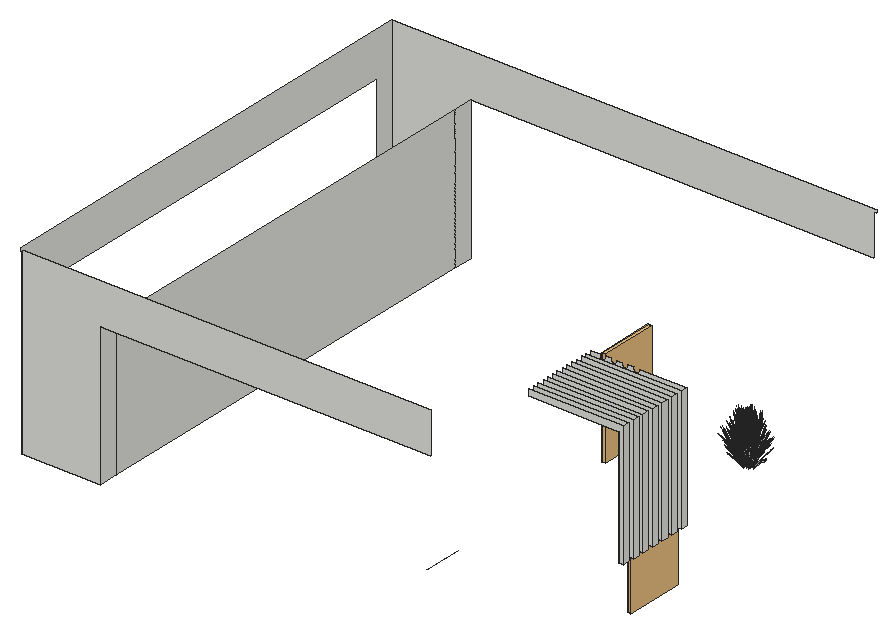
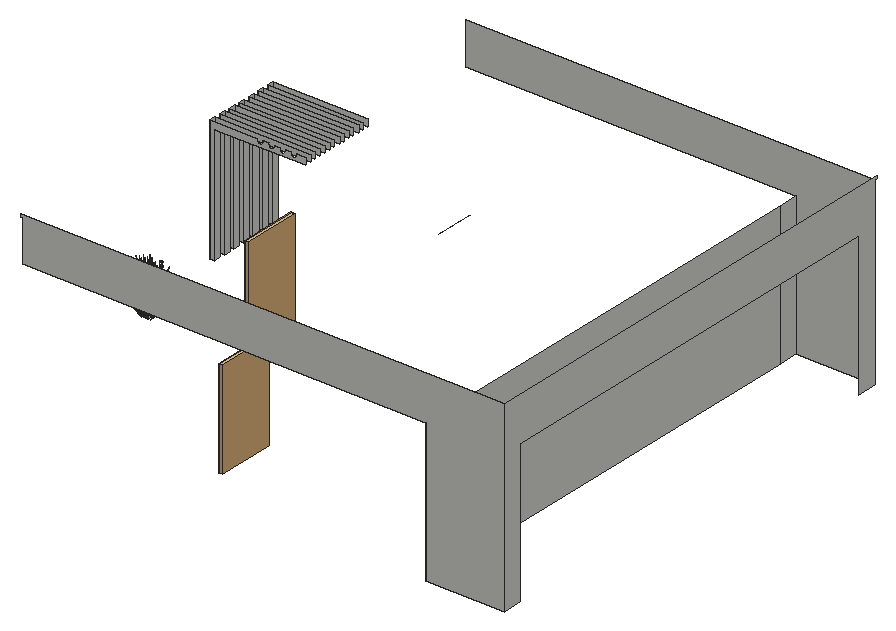
# SketchUp Ruby script. Lengths in millimetres.
U = 1.mm
M = Sketchup.active_model
def pt(a) = Geom::Point3d.new(a.map { |v| v * U })
def face(e, loops, mat)
  f = e.add_face(loops[0].map { |a| pt(a) })
  loops[1..].each { |l| e.add_face(l.map { |a| pt(a) }).erase! }
  f.material = f.back_material = mat if mat
  f
end
# faces: each face lists its corners as indices into pts; further lists are holes
def faces(e, pts, list, mat = nil) = list.each { |f| face(e, (f[0].is_a?(Array) ? f : [f]).map { |l| l.map { |i| pts[i] } }, mat) }
# xy, xz, yz: faces in a plane at the given z, y or x. An outline is a flat list of corners, or four numbers for a rectangle; further outlines are holes
def ring(l) = l.size == 4 ? [[l[0], l[1]], [l[2], l[1]], [l[2], l[3]], [l[0], l[3]]] : l.each_slice(2).to_a
def flat(e, list, mat, &to3) = list.each { |f| face(e, (f[0].is_a?(Array) ? f : [f]).map { |l| ring(l).map { |u, v| to3.(u, v) } }, mat) }
def xy(e, z, list, mat = nil) = flat(e, list, mat) { |x, y| [x, y, z] }
def xz(e, y, list, mat = nil) = flat(e, list, mat) { |x, z| [x, y, z] }
def yz(e, x, list, mat = nil) = flat(e, list, mat) { |y, z| [x, y, z] }
def lines(e, pts, list) = list.each { |a, b| e.add_line(pt(pts[a]), pt(pts[b])) }
# prism: a flat outline (further loops are holes) pulled along v
def prism(e, loops, v, mat = nil)
  f = face(e, loops, mat); d = Geom::Vector3d.new(v.map { |x| x * U })
  f.pushpull(f.normal.samedirection?(d) ? d.length : -d.length)
end
def box(e, o, s, mat = nil) = prism(e, [[o, [o[0] + s[0], o[1], o[2]], [o[0] + s[0], o[1] + s[1], o[2]], [o[0], o[1] + s[1], o[2]]]], [0, 0, s[2]], mat)
def at(x, y, z, deg = 0) = Geom::Transformation.translation(pt([x, y, z])) * Geom::Transformation.rotation(ORIGIN, Z_AXIS, deg.degrees)
def axes(o, x, y, z) = Geom::Transformation.new([*x, 0, *y, 0, *z, 0, *pt(o).to_a, 1])
def part(name) = M.definitions.add(name)
# library, detail: a bought-in or finely detailed component or shape, given as its bounding box
def library(name, o, s) = part(name).tap { |d| box(d.entities, o, s) }
def detail(e, o, s) = box(e.add_group.entities, o, s)
def put(e, d, t, mat = nil) = e.add_instance(d, t).tap { |i| i.material = mat if mat }
def group(e, t, mat = nil) = e.add_group.tap { |g| g.transformation = t; g.material = mat if mat }.entities
root = M.entities
M.materials.add("LightPink_Translucent").color = [144, 107, 117]
M.materials["LightPink_Translucent"].alpha = 0.8
c1 = library("porta+4",[5.1,-137.5,33.9],[1182.3,119.8,2113.3])
c2 = part("blade")
p = [[54.7,5.3,558.8],[0,4.4,0],[2.3,11.5,0],[55.5,7.8,558.8],[58.2,7.8,558.8],[9.8,11.5,0],
  [62.9,5.7,838.2],[63,6,838.2],[63.4,6,838.2]]
faces(c2.entities,p,[[0,1,2,3],[4,5,2,3],[6,0,3,7],[7,3,4,8]])
c3 = part("seeds")
p = [[7.6,-2.7,35.1],[-0.2,-0.6,40.4],[-0.2,-0.8,0.9],[3.5,-1.8,-1.7],[7.5,-0.8,76.3],[3.7,0.2,78.9]]
faces(c3.entities,p,[[0,1,2,3],[1,0,4,5]],"LightPink_Translucent")
c4 = part("blade with seeds")
put(c4.entities,c2,at(0,0,0))
put(c4.entities,c3,axes([60.9,6.5,787.2],[1.5799,-0.05474,1.17369],[-0.12525,1.92788,0.29478],[-0.07173,-0.02425,1.56792]))
xy(root,8077.2,[[16840.2,7010.7,16992.6,7213.9],[16840.2,7383.7,16992.6,7586.9],[16840.2,7756.7,16992.6,7959.9],[16840.2,8129.7,16992.6,8332.9],[16840.2,8502.7,16992.6,8705.9],
  [16840.2,8875.6,16992.6,9078.8],[16840.2,9248.6,16992.6,9449.1]])
xz(root,3200.4,[[1295.4,7315.2,3733.8,7315.2,3733.8,11734.8,14020.8,11734.8,14020.8,13030.2,1295.4,13030.2]])
xz(root,7010.7,[[16840.2,8077.2,16992.6,8077.2,16992.6,11938,14020.8,11938,14020.8,11734.8,16840.2,11734.8]])
xz(root,7213.9,[[16840.2,8077.2,16840.2,11734.8,14020.8,11734.8,14020.8,11938,16992.6,11938,16992.6,8077.2]])
xz(root,7383.7,[[16840.2,8077.2,16992.6,8077.2,16992.6,11938,14020.8,11938,14020.8,11734.8,16840.2,11734.8]])
xz(root,7586.9,[[16840.2,8077.2,16840.2,11734.8,14020.8,11734.8,14020.8,11938,16992.6,11938,16992.6,8077.2]])
xz(root,7756.7,[[16840.2,8077.2,16992.6,8077.2,16992.6,11938,14020.8,11938,14020.8,11734.8,16840.2,11734.8]])
xz(root,7959.9,[[16840.2,8077.2,16840.2,11734.8,14020.8,11734.8,14020.8,11938,16992.6,11938,16992.6,8077.2]])
xz(root,8129.7,[[16840.2,8077.2,16992.6,8077.2,16992.6,11938,14020.8,11938,14020.8,11734.8,16840.2,11734.8]])
xz(root,8332.9,[[16840.2,8077.2,16840.2,11734.8,14020.8,11734.8,14020.8,11938,16992.6,11938,16992.6,8077.2]])
xz(root,8502.7,[[16840.2,8077.2,16992.6,8077.2,16992.6,11938,14020.8,11938,14020.8,11734.8,16840.2,11734.8]])
xz(root,8705.9,[[16840.2,8077.2,16840.2,11734.8,14020.8,11734.8,14020.8,11938,16992.6,11938,16992.6,8077.2]])
xz(root,8875.6,[[16840.2,8077.2,16992.6,8077.2,16992.6,11938,14020.8,11938,14020.8,11734.8,16840.2,11734.8]])
xz(root,9078.8,[[16840.2,8077.2,16840.2,11734.8,14020.8,11734.8,14020.8,11938,16992.6,11938,16992.6,8077.2]])
xz(root,9248.6,[[16840.2,8077.2,16992.6,8077.2,16992.6,11938,14020.8,11938,14020.8,11734.8,16840.2,11734.8]])
xz(root,9449.1,[[16840.2,8077.2,16840.2,11734.8,14020.8,11734.8,14020.8,11938,14283.3,11938,14279.8,11929.5,14276.3,11903.2,14279.8,11876.9,14290,11852.4,14306.1,11831.4,14327.1,11815.3,14351.7,11805.1,14377.9,11801.6,14404.2,11805.1,14428.7,11815.3,14449.8,11831.4,14465.9,11852.4,14476.1,11876.9,14479.5,11903.2,14476.1,11929.5,14472.6,11938,14637.6,11938,14634.1,11929.5,14630.7,11903.2,14634.1,11876.9,14644.3,11852.4,14660.4,11831.4,14681.5,11815.3,14706,11805.1,14732.3,11801.6,14758.6,11805.1,14783.1,11815.3,14804.1,11831.4,14820.2,11852.4,14830.4,11876.9,14833.9,11903.2,14830.4,11929.5,14826.9,11938,14985.8,11938,14982.3,11929.5,14978.9,11903.2,14982.3,11876.9,14992.5,11852.4,15008.6,11831.4,15029.7,11815.3,15054.2,11805.1,15080.5,11801.6,15106.8,11805.1,15131.3,11815.3,15152.3,11831.4,15168.4,11852.4,15178.6,11876.9,15182.1,11903.2,15178.6,11929.5,15175.1,11938,15337.8,11938,15334.3,11929.5,15330.8,11903.2,15334.3,11876.9,15344.4,11852.4,15360.6,11831.4,15381.6,11815.3,15406.1,11805.1,15432.4,11801.6,15458.7,11805.1,15483.2,11815.3,15504.2,11831.4,15520.4,11852.4,15530.5,11876.9,15534,11903.2,15530.5,11929.5,15527,11938,16992.6,11938,16992.6,8077.2]])
xz(root,17602.2,[[1295.4,7315.2,1295.4,13106.4,16383,13106.4,16383,13030.2,16306.8,13030.2,16306.8,11734.8,3733.8,11734.8,3733.8,7315.2]])
yz(root,1295.4,[[3200.4,7315.2,3200.4,13030.2,3124.2,13030.2,3124.2,13106.4,17602.2,13106.4,17602.2,7315.2,16992.6,7315.2,16992.6,11734.8,3810,11734.8,3810,7315.2]])
yz(root,3733.8,[[3200.4,7315.2,3810,11734.8],[3810,7315.2,16992.6,11734.8],[16992.6,7315.2,17602.2,11734.8]])
yz(root,16840.2,[[7010.7,8077.2,7213.9,11734.8],[7383.7,8077.2,7586.9,11734.8],[7756.7,8077.2,7959.9,11734.8],[8129.7,8077.2,8332.9,11734.8],[8502.7,8077.2,8705.9,11734.8],
  [8875.6,8077.2,9078.8,11734.8],[9248.6,8077.2,9449.1,11734.8]])
yz(root,16992.6,[[7010.7,8077.2,7213.9,11938],[7383.7,8077.2,7586.9,11938],[7756.7,8077.2,7959.9,11938],[8129.7,8077.2,8332.9,11938],[8502.7,8077.2,8705.9,11938],
  [8875.6,8077.2,9078.8,11938],[9248.6,8077.2,9449.1,11938]])
p = [[13411.2,5029.2,8077.2],[13411.2,3810,8077.2],[3733.8,3810,7315.2],[3733.8,3810,7314.8]]
lines(root,p,[[0,1],[2,3]])
put(root,c1,axes([14278.9,10507.8,4216.9],[0,1.53,0],[-1,0,0],[0,0,1.44274]))
put(root,c1,axes([13364.5,10646.4,8026.9],[0,1.53,0],[-1,0,0],[0,0,1.44274]))
put(root,c4,axes([16282.1,12651.4,8130.5],[-0.50328,-1.06202,-0.69835],[1.44974,-0.38248,-0.18329],[-0.05563,-0.35963,1.54149]))
put(root,c4,axes([16399,12697.2,8130.4],[0.44936,0.94823,-0.69212],[-1.29441,0.3415,-0.18165],[0.04967,0.32109,1.52773]))
put(root,c4,axes([16395.7,12646.7,8129.5],[1.27479,0.1698,-0.62353],[-0.26901,1.04736,-0.16365],[0.38043,0.12691,1.37633]))
put(root,c4,axes([16287.1,12701.7,8129.5],[-1.27479,-0.1698,-0.62353],[0.26901,-1.04736,-0.16365],[-0.38043,-0.12691,1.37633]))
put(root,c4,axes([16338,12623.7,8129.5],[0.82544,-0.77843,-0.62353],[1.0254,0.70586,-0.16365],[0.33076,-0.19418,1.37633]))
put(root,c4,axes([16344.7,12724.8,8129.5],[-0.82544,0.77843,-0.62353],[-1.0254,-0.70586,-0.16365],[-0.33076,0.19418,1.37633]))
put(root,c4,axes([16438.1,12596.4,8128.4],[1.14694,0.51783,-0.49651],[-0.68554,0.92854,0],[0.26122,0.11794,1.57504]))
put(root,c4,axes([16379.2,12778.7,8128.4],[-1.14694,0.51783,-0.49651],[-0.68554,-0.92854,0],[-0.26122,0.11794,1.57504]))
put(root,c4,axes([16206.8,12647.6,8128.4],[0,-1.03566,-0.49651],[1.37109,0,0],[0,-0.23588,1.57504]))
put(root,c4,axes([16244.6,12752.1,8128.4],[-1.14694,-0.51783,-0.49651],[0.68554,-0.92854,0],[-0.26122,-0.11794,1.57504]))
put(root,c4,axes([16303.5,12569.8,8128.4],[1.14694,-0.51783,-0.49651],[0.68554,0.92854,0],[0.26122,-0.11794,1.57504]))
put(root,c4,axes([16476,12700.8,8128.4],[0,1.03566,-0.49651],[-1.37109,0,0],[0,0.23588,1.57504]))
put(root,c4,axes([16301.5,12658.4,8133.4],[0.59459,-0.93321,-0.44739],[1.23546,0.44912,0.21531],[0,-0.21512,1.43643]))
put(root,c4,axes([16303.9,12693.3,8133.4],[-0.73619,-0.86927,-0.44739],[1.11511,-0.61213,0.21531],[-0.23824,-0.10756,1.43643]))
put(root,c4,axes([16378.9,12655.2,8133.4],[0.73619,0.86927,-0.44739],[-1.11511,0.61213,0.21531],[0.23824,0.10756,1.43643]))
put(root,c4,axes([16381.2,12690.1,8133.4],[-0.59459,0.93321,-0.44739],[-1.23546,-0.44912,0.21531],[0,0.21512,1.43643]))
put(root,c4,axes([16343.7,12709.1,8133.4],[-1.33077,0.06393,-0.44739],[-0.12035,-1.06125,0.21531],[-0.23824,0.10756,1.43643]))
put(root,c4,axes([16310.3,12580.2,8128.7],[1.14332,0.25625,-0.30978],[-0.28787,0.90242,0.30978],[0.23049,-0.10406,1.38974]))
put(root,c4,axes([16461.1,12700.3,8128.7],[-0.85545,0.64616,-0.30978],[-0.85545,-0.64616,0.30978],[0,0.20813,1.38974]))
put(root,c4,axes([16252.7,12742.3,8128.7],[-0.28787,-0.90242,-0.30978],[1.14332,-0.25625,0.30978],[-0.23049,-0.10406,1.38974]))
put(root,c4,axes([16372.4,12768.3,8128.7],[-1.14332,-0.25625,-0.30978],[0.28787,-0.90242,0.30978],[-0.23049,0.10406,1.38974]))
put(root,c4,axes([16430,12606.2,8128.7],[0.28787,0.90242,-0.30978],[-1.14332,0.25625,0.30978],[0.23049,0.10406,1.38974]))
put(root,c4,axes([16221.7,12648.2,8128.7],[0.85545,-0.64616,-0.30978],[0.85545,0.64616,0.30978],[0,-0.20813,1.38974]))
put(root,c4,axes([16436.7,12783.5,8115.1],[0.08928,-0.14952,1.76342],[1.12407,-0.44035,-0.26939],[0.34078,0.22791,0.30037]))
put(root,c4,axes([16183,12664.2,8115.1],[0.03108,0.16322,1.76342],[-0.62654,0.85237,-0.26939],[-0.44504,-0.04296,0.30037]))
put(root,c4,axes([16325.2,12523.6,8115.1],[-0.20555,0.03731,1.76342],[-1.13672,-0.42002,-0.26939],[0.01907,-0.35034,0.30037]))
put(root,c4,axes([16303.3,12782.7,8115.1],[0.19833,-0.05635,1.76342],[1.19302,0.31018,-0.26939],[0.03489,0.3496,0.30037]))
put(root,c4,axes([16518.9,12668.2,8115.1],[-0.06405,-0.15723,1.76342],[0.44421,-0.91974,-0.26939],[0.4481,-0.01323,0.30037]))
put(root,c4,axes([16231.8,12556.2,8115.1],[-0.11871,0.13643,1.76342],[-1.19964,0.29415,-0.26939],[-0.2898,-0.26759,0.30037]))
put(root,c4,axes([16174.5,12780.3,8115.1],[0.16438,0.10347,1.76342],[0.27873,0.95868,-0.26939],[-0.36432,0.20444,0.30037]))
put(root,c4,axes([16453,12569,8115.1],[-0.18342,-0.08159,1.76342],[-0.47115,-0.9115,-0.26939],[0.31784,-0.24736,0.30037]))
put(root,c4,axes([16279.6,12627.2,8117.7],[-1.20625,0.41464,1.28929],[-0.38394,-1.1897,0.50096],[0.74071,0.01979,1.46642]))
put(root,c4,axes([16367.4,12701.8,8144.9],[0.1428,1.18174,-0.29095],[-1.48733,0.07145,-0.50002],[-0.26191,0.15741,1.59708]))
put(root,c4,axes([16385,12670.4,8144.9],[1.38012,0.49416,-0.29095],[-0.66454,1.04299,-0.50002],[0.04337,0.25608,1.59708]))
put(root,c4,axes([16297.8,12678.1,8144.9],[-1.38012,-0.49416,-0.29095],[0.66454,-1.04299,-0.50002],[-0.04337,-0.25608,1.59708]))
put(root,c4,axes([16315.3,12646.6,8144.9],[-0.1428,-1.18174,-0.29095],[1.48733,-0.07145,-0.50002],[0.26191,-0.15741,1.59708]))
put(root,c4,axes([16358.9,12642.8,8144.9],[1.23732,-0.68758,-0.29095],[0.8228,0.97154,-0.50002],[0.30528,0.09867,1.59708]))
put(root,c4,axes([16323.8,12705.7,8144.9],[-1.23732,0.68758,-0.29095],[-0.8228,-0.97154,-0.50002],[-0.30528,-0.09867,1.59708]))
put(root,c4,axes([16378.2,12731.6,8132.7],[1.2866,-0.3514,-0.19198],[0.45209,1.01223,0.00008],[0.14202,-0.03884,1.73897]))
put(root,c4,axes([16359.1,12713.6,8139.8],[-1.19666,-0.83357,-0.25192],[1.00694,-0.93603,0.5513],[-0.32224,0.09751,1.68216]))
put(root,c4,axes([16306.6,12706,8139.1],[0.32481,-1.2272,-0.23429],[1.54007,0.21392,0.51271],[-0.26911,-0.16947,1.5644]))
put(root,c4,axes([16319.8,12542.1,8131.3],[-0.84686,0.59414,-0.03893],[-0.77596,-0.65071,-0.17649],[-0.05463,-0.18438,0.58215]))
put(root,c4,axes([16212.9,12569.5,8131.3],[-0.35352,0.84566,-0.03893],[-1.08806,-0.26014,-0.17649],[-0.1652,-0.13832,0.58215]))
put(root,c4,axes([16533.5,12662.4,8134.6],[-0.75977,-0.66224,-0.06488],[0.83212,-0.6068,-0.29416],[0.23578,-0.04272,0.97024]))
put(root,c4,axes([16497,12684.7,8127.6],[-0.7893,0.12429,1.41583],[-0.12563,-0.9893,0.08104],[0.55282,-0.14974,0.80566]))
put(root,c4,axes([16381.2,12771.7,8132.9],[-0.75665,-1.04141,-0.05142],[1.28187,-0.57875,0.51607],[-0.31588,0.09915,1.6363]))
put(root,c4,axes([16469.2,12696,8133.1],[-1.53164,-0.00828,-0.04976],[0,-1.1575,0.49943],[-0.04813,0.2635,1.58352]))
put(root,c4,axes([16357.4,12735.6,8135.4],[0.53281,1.18979,-0.06012],[-1.52239,0.41691,0],[0.01861,0.04155,1.72173]))
put(root,c4,axes([16366.2,12688.2,8135.6],[-1.1399,-0.8914,-0.06131],[1.1406,-0.89194,0],[-0.03981,-0.03113,1.75571]))
put(root,c4,axes([16376,12676.8,8135.4],[0,1.19774,-0.05637],[-1.53239,0,0],[0,0.03764,1.79368]))
put(root,c4,axes([16277.1,12573.9,8137.5],[-0.7662,-1.03778,0],[1.28187,-0.57875,-0.51607],[0.29196,-0.13181,1.63711]))
put(root,c4,axes([16262.3,12768,8137.5],[-0.7662,1.03778,0],[-1.28187,-0.57875,-0.51607],[-0.29196,-0.13181,1.63711]))
put(root,c4,axes([16405.7,12774.6,8137.5],[0.7662,1.03778,0],[-1.28187,0.57875,-0.51607],[-0.29196,0.13181,1.63711]))
put(root,c4,axes([16198,12667.6,8137.5],[-1.53239,0,0],[0,-1.1575,-0.51607],[0,-0.26363,1.63711]))
put(root,c4,axes([16420.4,12580.5,8137.6],[0.7662,-1.03778,0],[1.28187,0.57875,-0.51607],[0.29196,0.13181,1.63711]))
put(root,c4,axes([16484.7,12680.9,8137.6],[1.53239,0,0],[0,1.1575,-0.51607],[0,0.26363,1.63711]))
put(root,c4,axes([16228.2,12659.8,8136.4],[-1.1399,0.87071,0.30756],[-1.1406,-0.86155,-0.36492],[-0.03981,-0.24727,1.64885]))
put(root,c4,axes([16382,12758.1,8136.4],[1.53422,0.33662,0.30756],[-0.38383,1.20322,-0.36492],[-0.25393,0.15059,1.64885]))
put(root,c4,axes([16333.1,12745.1,8133],[-1.23546,-0.46496,0],[0.59459,-0.96613,0],[0,0,1.62707]))
put(root,c4,axes([16368.7,12745.5,8133.2],[1.23546,0.46496,0],[-0.59459,0.96613,0],[0,0,1.74954]))
put(root,c4,axes([16340.2,12734.8,8133.2],[-0.39985,-0.89288,0],[1.1418,-0.31268,0],[0,0,1.54371]))
put(root,c4,axes([16356.4,12664.6,8133.2],[0,-1.19833,0],[1.53239,0,0],[0,0,1.79456]))
put(root,c4,axes([16382.8,12671.4,8133.2],[1.37109,0,0],[0,1.07219,0],[0,0,1.78407]))
put(root,c4,axes([16382.1,12683.1,8133.4],[0.85545,0.66896,0],[-0.85545,0.66896,0],[0,0,1.69266]))
put(root,c4,axes([16311.1,12690.9,8137.2],[1.54892,0.2182,0.45755],[-0.31522,1.23236,0.17955],[-0.22636,-0.119,1.58856]))
put(root,c4,axes([16338,12645.4,8137.2],[-1.01611,0.93987,0.45755],[-1.20717,-0.82966,0.17955],[0.24496,-0.0938,1.58856]))
put(root,c4,axes([16307.8,12662.1,8137.2],[0.53281,1.15808,0.45755],[-1.52239,0.4027,0.17955],[0.01861,-0.2128,1.58856]))
put(root,c4,axes([16371.6,12657.5,8137.7],[-1.54892,-0.2182,0.49198],[0.31522,-1.23236,0.19306],[0.22636,0.119,1.70813]))
put(root,c4,axes([16320.3,12670.2,8139],[1.3808,0.50196,0.24065],[-0.66454,1.04299,0.50002],[0,-0.24043,1.60543]))
put(root,c4,axes([16374.4,12707.7,8143.7],[0.90538,0.62224,0.1448],[-0.75521,0.70202,-0.41347],[-0.21021,0.09491,1.26744]))
put(root,c4,axes([16361.9,12635.2,8143.7],[0.23642,-0.92427,0.1448],[1.15506,0.16044,-0.41347],[0.21021,0.09491,1.26744]))
put(root,c4,axes([16394.9,12668.6,8143.7],[1.1418,-0.30203,0.1448],[0.39985,0.86246,-0.41347],[0,0.18981,1.26744]))
put(root,c4,axes([16320.8,12713.3,8143.7],[-0.23642,0.92427,0.1448],[-1.15506,-0.16044,-0.41347],[-0.21021,-0.09491,1.26744]))
put(root,c4,axes([16233.7,12786.2,8148.9],[1.11329,-0.1834,0.06507],[0.25594,0.73887,-0.86304],[-0.07058,0.37403,0.7736]))
put(root,c4,axes([16204.7,12615.1,8143],[0.23927,0.28834,1.43002],[-0.55135,0.78376,-0.30754],[-0.56612,-0.18733,0.61141]))
put(root,c4,axes([16226.8,12806.2,8143],[0.38672,-0.16338,1.43002],[0.95481,0.49262,-0.30754],[-0.28419,0.42626,0.61141]))
put(root,c4,axes([16369.4,12747.3,8143],[0.02163,-0.34331,1.43002],[1.03345,-0.38348,-0.30754],[0.31903,0.4109,0.61141]))
put(root,c4,axes([16391.1,12552.5,8143],[-0.34835,0.20963,1.43002],[-1.04325,-0.36691,-0.30754],[0.19338,-0.4563,0.61141]))
put(root,c4,axes([16476.4,12615.2,8143],[-0.4378,-0.03068,1.43002],[-0.44851,-0.8229,-0.30754],[0.53783,-0.23279,0.61141]))
put(root,c4,axes([16254.2,12542.5,8143],[-0.07421,0.33879,1.43002],[-1.08488,0.28361,-0.30754],[-0.25359,-0.4379,0.61141]))
put(root,c4,axes([16502.7,12722,8143],[-0.29514,-0.25472,1.43002],[0.38401,-0.84262,-0.30754],[0.59714,0.11414,0.61141]))
put(root,c4,axes([16162.9,12721.8,8143],[0.42589,0.08502,1.43002],[0.2745,0.86839,-0.30754],[-0.57851,0.16255,0.61141]))
put(root,c4,axes([16392.7,12607.5,8140],[-1.31687,0.27488,0.17642],[-0.32517,-1.02297,0.35086],[0.11745,0.14905,1.60407]))
put(root,c4,axes([16440.9,12675.7,8140],[-0.96285,-0.75439,0.17642],[0.97031,-0.7317,0.35086],[-0.10634,0.15406,1.60407]))
put(root,c4,axes([16293.2,12606.1,8140],[-0.35402,1.02926,0.17642],[-1.29548,-0.29127,0.35086],[0.22379,-0.00501,1.60407]))
put(root,c4,axes([16389.6,12742.4,8140],[0.35402,-1.02926,0.17642],[1.29548,0.29127,0.35086],[-0.22379,0.00501,1.60407]))
put(root,c4,axes([16290,12740.9,8140],[1.31687,-0.27488,0.17642],[0.32517,1.02297,0.35086],[-0.11745,-0.14905,1.60407]))
put(root,c4,axes([16221.7,12672.1,8140.2],[0,1.03566,0.49651],[-1.37109,0,0],[0,-0.23588,1.57504]))
put(root,c4,axes([16403.6,12594.3,8140.2],[-1.14694,-0.51783,0.49651],[0.68554,-0.92854,0],[0.26122,0.11794,1.57504]))
put(root,c4,axes([16461.1,12676.4,8140.2],[0,-1.03566,0.49651],[1.37109,0,0],[0,0.23588,1.57504]))
put(root,c4,axes([16398.8,12756.4,8140.2],[1.14694,-0.51783,0.49651],[0.68554,0.92854,0],[-0.26122,0.11794,1.57504]))
put(root,c4,axes([16279.1,12754.2,8140.2],[1.14694,0.51783,0.49651],[-0.68554,0.92854,0],[-0.26122,-0.11794,1.57504]))
put(root,c4,axes([16381.8,12663.2,8146.2],[0.59459,-0.93321,0.44739],[1.23546,0.44912,-0.21531],[0,0.21512,1.43643]))
put(root,c4,axes([16308.9,12652.4,8146.2],[-1.33077,0.06393,0.44739],[-0.12035,-1.06125,-0.21531],[0.23824,-0.10756,1.43643]))
put(root,c4,axes([16349.3,12641.4,8146.2],[-0.73619,-0.86927,0.44739],[1.11511,-0.61213,-0.21531],[0.23824,0.10756,1.43643]))
put(root,c4,axes([16301,12685.3,8146.2],[-0.59459,0.93321,0.44739],[-1.23546,-0.44912,-0.21531],[0,-0.21512,1.43643]))
put(root,c4,axes([16373.8,12696.1,8146.2],[1.33077,-0.06393,0.44739],[0.12035,1.06125,-0.21531],[-0.23824,0.10756,1.43643]))
put(root,c4,axes([16434.6,12789.8,8144.9],[-0.78586,-0.03248,1.0506],[0.51898,-0.68985,0.58006],[0.31045,0.24509,0.8241]))
put(root,c4,axes([16168.5,12637.1,8147.4],[0.78239,-0.07411,1.1486],[-0.49629,0.65296,0.84392],[-0.38663,-0.09795,0.25299]))
put(root,c4,axes([16431.8,12755.4,8147.4],[-0.69001,-0.29779,1.1486],[0.89096,-0.30257,0.84392],[0.24031,0.2563,0.25299]))
put(root,c4,axes([16140.3,12768,8147.4],[0.51072,-0.46938,1.1486],[0.20153,0.74307,0.84392],[-0.36908,0.13305,0.25299]))
put(root,c4,axes([16538.7,12693.2,8147.4],[-0.75718,0.17097,1.1486],[0.35641,-0.70661,0.84392],[0.40168,0.04835,0.25299]))
put(root,c4,axes([16244.7,12528.6,8147.4],[0.63926,0.36046,1.1486],[-0.93099,0.21668,0.84392],[-0.1992,-0.27702,0.25299]))
put(root,c4,axes([16250.3,12820,8147.4],[-0.03171,-0.6158,1.1486],[0.7925,0.43922,0.84392],[-0.15586,0.29352,0.25299]))
put(root,c4,axes([16489.2,12576.8,8147.4],[-0.40819,0.5272,1.1486],[-0.35086,-0.70831,0.84392],[0.33713,-0.17749,0.25299]))
put(root,c4,axes([16358.6,12510.2,8147.4],[0.15721,0.60392,1.1486],[-0.87211,-0.33448,0.84392],[0.09385,-0.30923,0.25299]))
put(root,c4,axes([16389.1,12670.3,8149.4],[-0.03348,-0.97511,1.41272],[1.51511,0.25277,0.59816],[-0.35835,0.53357,1.3335]))
put(root,c4,axes([16283.9,12577.1,8203.7],[-1.04497,-0.50058,-0.71045],[0.74264,-0.8772,0.08574],[-0.3786,-0.29889,1.00501]))
put(root,c4,axes([16312.8,12772.5,8203.7],[0.5849,0.8421,-0.71045],[-1.20401,0.4693,0.08574],[0.13677,0.40688,1.00501]))
put(root,c4,axes([16229.8,12608.6,8203.7],[-1.22504,-0.02494,-0.71045],[0.08228,-1.05005,0.08574],[-0.51899,-0.11081,1.00501]))
put(root,c4,axes([16452.9,12634.3,8203.7],[0.64013,-0.81717,-0.71045],[1.12174,0.58074,0.08574],[0.38221,-0.29607,1.00501]))
put(root,c4,axes([16460.6,12686.6,8203.7],[1.07686,-0.45739,-0.71045],[0.60013,0.94154,0.08574],[0.52031,-0.10696,1.00501]))
put(root,c4,axes([16412.7,12592,8203.7],[0.03189,-0.95798,-0.71045],[1.34277,0.06434,0.08574],[0.14171,-0.40585,1.00501]))
put(root,c4,axes([16433.9,12735,8203.7],[1.22504,0.02494,-0.71045],[-0.08228,1.05005,0.08574],[0.51899,0.11081,1.00501]))
put(root,c4,axes([16350.8,12571.1,8203.7],[-0.5849,-0.8421,-0.71045],[1.20401,-0.4693,0.08574],[-0.13677,-0.40688,1.00501]))
put(root,c4,axes([16324,12776.8,8196.1],[1.20468,0.25962,-0.51099],[-0.41292,0.89013,-0.3958],[0.11046,0.35838,0.97773]))
put(root,c4,axes([16405.8,12583.9,8196.1],[-0.87728,-0.69587,-0.51099],[0.92674,-0.60943,-0.3958],[0.13348,-0.35356,0.97773]))
put(root,c4,axes([16271.5,12577.8,8196.1],[-1.20928,0.24619,-0.51099],[-0.21154,-0.93233,-0.3958],[-0.32481,-0.26718,0.97773]))
put(root,c4,axes([16466.1,12677.9,8196.1],[0.332,-0.94205,-0.51099],[1.13828,0.3229,-0.3958],[0.45829,-0.08638,0.97773]))
put(root,c4,axes([16219.4,12614,8196.1],[-0.88986,0.68603,-0.51099],[-0.77932,-0.72471,-0.3958],[-0.45212,-0.10438,0.97773]))
put(root,c4,axes([16211.6,12719,8196.1],[0.31482,0.94565,-0.51099],[-1.19224,0.16542,-0.3958],[-0.34166,0.254,0.97773]))
put(root,c4,axes([16197.5,12665.7,8196.1],[-0.332,0.94205,-0.51099],[-1.13828,-0.3229,-0.3958],[-0.45829,0.08638,0.97773]))
put(root,c4,axes([16339.7,12566.8,8196.1],[-1.20468,-0.25962,-0.51099],[0.41292,-0.89013,-0.3958],[-0.11046,-0.35838,0.97773]))
put(root,c4,axes([16452,12624.6,8196.1],[-0.31482,-0.94565,-0.51099],[1.19224,-0.16542,-0.3958],[0.34166,-0.254,0.97773]))
put(root,c4,axes([16392.2,12765.8,8196.1],[1.20928,-0.24619,-0.51099],[0.21154,0.93233,-0.3958],[0.32481,0.26718,0.97773]))
put(root,c4,axes([16251,12751.6,8212.8],[-0.03189,0.95798,-0.7886],[-1.34277,-0.06434,0.09517],[-0.14171,0.40585,1.11556]))
put(root,c4,axes([16257.9,12759.7,8204.3],[0.87728,0.69587,-0.5672],[-0.92674,0.60943,-0.43934],[-0.13348,0.35356,1.08528]))
put(root,c4,axes([16347.4,12721,8161.7],[1.05902,0.41762,1.51261],[-1.03748,0.89969,0.59816],[-0.46471,-0.53324,1.26806]))
put(root,c4,axes([16258.6,12651.2,8162.1],[0.34834,-0.14982,1.77064],[0.12012,1.04605,0.13857],[-0.75452,0.1388,0.63284]))
put(root,c4,axes([16239.5,12785.9,8162.6],[0.02693,-0.53464,1.54345],[1.21102,0.2824,0.21329],[-0.10493,0.5698,0.72882]))
put(root,c4,axes([16452.6,12746,8192.2],[0.69728,0.64842,-0.35414],[-0.79619,0.61382,0.4572],[0.40453,0.09339,0.87481]))
put(root,c4,axes([16179.8,12654.7,8192.2],[-1.01846,-0.28891,-0.35414],[0.29705,-0.84289,0.4572],[-0.41005,0.07729,0.87481]))
put(root,c4,axes([16189.2,12716.5,8192.2],[-1.06674,0.14801,-0.35414],[-0.28168,-0.84611,0.4572],[-0.30569,0.22726,0.87481]))
put(root,c4,axes([16483.8,12688.8,8192.2],[1.01846,0.28891,-0.35414],[-0.29705,0.84289,0.4572],[0.41005,-0.07729,0.87481]))
put(root,c4,axes([16274.7,12560.3,8192.2],[-0.18927,-0.83419,-0.35414],[1.08199,-0.22027,0.4572],[-0.29062,-0.23905,0.87481]))
put(root,c4,axes([16236.9,12766.2,8192.2],[-0.82919,0.54528,-0.35414],[-0.78493,-0.62262,0.4572],[-0.11943,0.31634,0.87481]))
put(root,c4,axes([16474.4,12627.1,8192.2],[1.06674,-0.14801,-0.35414],[0.28168,0.84611,0.4572],[0.30569,-0.22726,0.87481]))
put(root,c4,axes([16310,12790.7,8192.2],[-0.36946,0.79643,-0.35414],[-1.07787,-0.23229,0.4572],[0.09883,0.32066,0.87481]))
put(root,c4,axes([16426.7,12577.4,8192.2],[0.82919,-0.54528,-0.35414],[0.78493,0.62262,0.4572],[0.11943,-0.31634,0.87481]))
put(root,c4,axes([16353.6,12552.9,8192.2],[0.36946,-0.79643,-0.35414],[1.07787,0.23229,0.4572],[-0.09883,-0.32066,0.87481]))
put(root,c4,axes([16211.1,12597.6,8192.2],[-0.69728,-0.64842,-0.35414],[0.79619,-0.61382,0.4572],[-0.40453,-0.09339,0.87481]))
put(root,c4,axes([16505.3,12748.5,8177],[-0.23455,-0.87059,-0.03492],[1.10861,-0.20015,-0.15832],[0.23151,0.05519,0.52218]))
put(root,c4,axes([16388.9,12703.8,8175.7],[-0.45521,-0.17844,1.71376],[0.94204,-0.74856,0.13857],[0.58713,0.33769,0.73262]))
put(root,c4,axes([16374.3,12579.7,8175.7],[-0.22818,0.35597,1.71376],[-0.95725,-0.73667,0.13857],[0.43183,-0.45914,0.73262]))
put(root,c4,axes([16413.4,12662.3,8175.7],[-0.50831,0.02346,1.71376],[0.33721,-1.01661,0.13857],[0.72439,0.06288,0.73262]))
put(root,c4,axes([16341.3,12730.1,8175.7],[-0.28013,-0.33252,1.71376],[1.29445,-0.27994,0.13857],[0.29256,0.52202,0.73262]))
put(root,c4,axes([16283.2,12734.3,8175.7],[-0.02999,-0.3975,1.71376],[1.30002,0.26369,0.13857],[-0.08041,0.56647,0.73262]))
put(root,c4,axes([16230.2,12715.2,8175.7],[0.22818,-0.35597,1.71376],[0.95725,0.73667,0.13857],[-0.43183,0.45914,0.73262]))
put(root,c4,axes([16196.5,12678,8175.7],[0.42521,-0.21906,1.71376],[0.35798,1.01226,0.13857],[-0.66754,0.22878,0.73262]))
put(root,c4,axes([16236,12695.3,8175.7],[0.30609,-0.31822,1.71376],[0.77286,0.85893,0.13857],[-0.53009,0.39116,0.73262]))
put(root,c4,axes([16263.2,12564.8,8175.7],[0.28013,0.33252,1.71376],[-1.29445,0.27994,0.13857],[-0.29256,-0.52202,0.73262]))
put(root,c4,axes([16215.6,12591.1,8175.7],[0.45521,0.17844,1.71376],[-0.94204,0.74856,0.13857],[-0.58713,-0.33769,0.73262]))
put(root,c4,axes([16191.1,12632.6,8175.7],[0.50831,-0.02346,1.71376],[-0.33721,1.01661,0.13857],[-0.72439,-0.06288,0.73262]))
